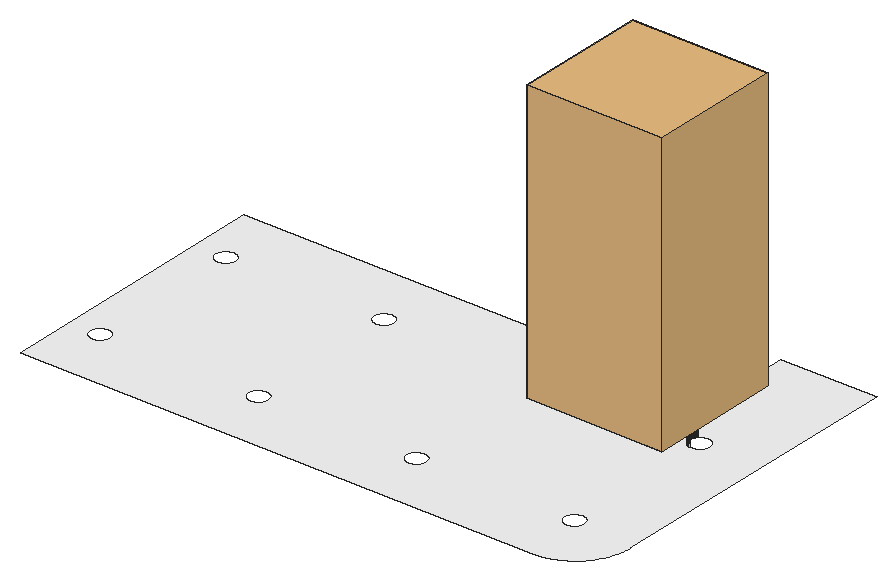
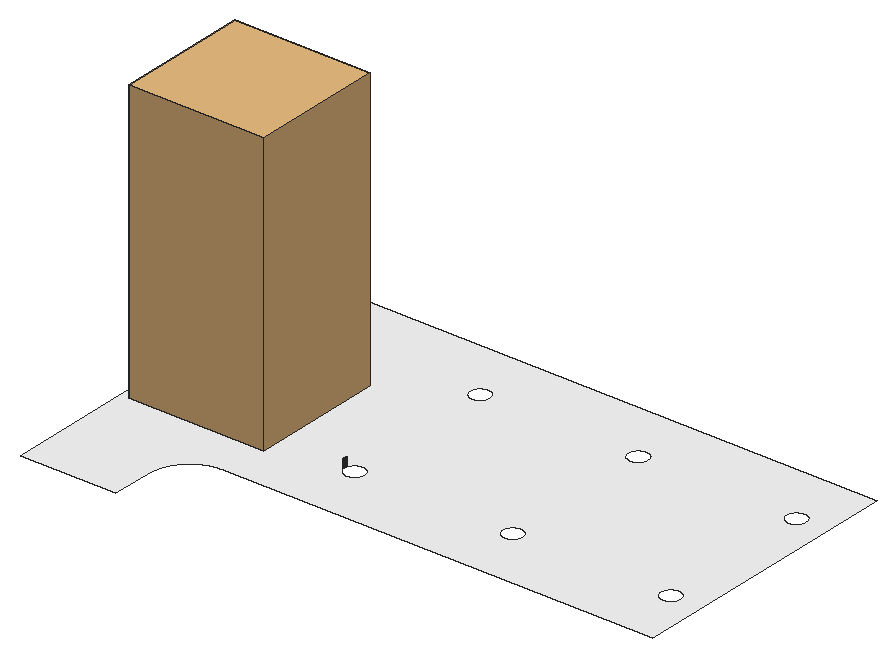
# SketchUp Ruby script. Lengths in inches.
U = 1.inch
M = Sketchup.active_model
def pt(a) = Geom::Point3d.new(a.map { |v| v * U })
def face(e, loops, mat)
  f = e.add_face(loops[0].map { |a| pt(a) })
  loops[1..].each { |l| e.add_face(l.map { |a| pt(a) }).erase! }
  f.material = f.back_material = mat if mat
  f
end
# faces: each face lists its corners as indices into pts; further lists are holes
def faces(e, pts, list, mat = nil) = list.each { |f| face(e, (f[0].is_a?(Array) ? f : [f]).map { |l| l.map { |i| pts[i] } }, mat) }
# xy, xz, yz: faces in a plane at the given z, y or x. An outline is a flat list of corners, or four numbers for a rectangle; further outlines are holes
def ring(l) = l.size == 4 ? [[l[0], l[1]], [l[2], l[1]], [l[2], l[3]], [l[0], l[3]]] : l.each_slice(2).to_a
def flat(e, list, mat, &to3) = list.each { |f| face(e, (f[0].is_a?(Array) ? f : [f]).map { |l| ring(l).map { |u, v| to3.(u, v) } }, mat) }
def xy(e, z, list, mat = nil) = flat(e, list, mat) { |x, y| [x, y, z] }
def xz(e, y, list, mat = nil) = flat(e, list, mat) { |x, z| [x, y, z] }
def yz(e, x, list, mat = nil) = flat(e, list, mat) { |y, z| [x, y, z] }
def lines(e, pts, list) = list.each { |a, b| e.add_line(pt(pts[a]), pt(pts[b])) }
# prism: a flat outline (further loops are holes) pulled along v
def prism(e, loops, v, mat = nil)
  f = face(e, loops, mat); d = Geom::Vector3d.new(v.map { |x| x * U })
  f.pushpull(f.normal.samedirection?(d) ? d.length : -d.length)
end
def box(e, o, s, mat = nil) = prism(e, [[o, [o[0] + s[0], o[1], o[2]], [o[0] + s[0], o[1] + s[1], o[2]], [o[0], o[1] + s[1], o[2]]]], [0, 0, s[2]], mat)
def at(x, y, z, deg = 0) = Geom::Transformation.translation(pt([x, y, z])) * Geom::Transformation.rotation(ORIGIN, Z_AXIS, deg.degrees)
def axes(o, x, y, z) = Geom::Transformation.new([*x, 0, *y, 0, *z, 0, *pt(o).to_a, 1])
def part(name) = M.definitions.add(name)
# library, detail: a bought-in or finely detailed component or shape, given as its bounding box
def library(name, o, s) = part(name).tap { |d| box(d.entities, o, s) }
def detail(e, o, s) = box(e.add_group.entities, o, s)
def put(e, d, t, mat = nil) = e.add_instance(d, t).tap { |i| i.material = mat if mat }
def group(e, t, mat = nil) = e.add_group.tap { |g| g.transformation = t; g.material = mat if mat }.entities
root = M.entities
M.materials.add("[Quartz Light Grey]").color = [251, 251, 252]
c1 = library("aaa (1)",[154.83,121.66,0],[39.67,38.89,82.21])
xy(root,117,[[[60,189,60,271,186.3125,271,186.47,271.01,186.63,271.02,186.78,271.03,187.1,271.05,187.25,271.07,187.41,271.08,187.57,271.1,187.72,271.125,187.88,271.15,188.03,271.17,188.1875,271.2,188.34,271.23,188.49,271.26,188.65,271.3,188.8,271.33,188.95,271.37,189.11,271.41,189.41,271.49,189.86,271.64,190.01,271.6875,190.15,271.74,190.3,271.8,190.45,271.85,190.59,271.91,190.74,271.97,190.88,272.04,191.02,272.1,191.17,272.17,191.73,272.45,191.86,272.53,192,272.61,192.14,272.6875,192.27,272.77,192.4,272.85,192.54,272.9375,192.67,273.02,192.93,273.2,193.05,273.29,193.18,273.38,193.31,273.48,193.43,273.58,193.55,273.67,193.67,273.77,193.91,273.98,194.03,274.08,194.15,274.1875,194.26,274.3,194.375,274.4,194.49,274.51,194.6,274.625,194.7,274.74,194.8125,274.85,194.92,274.97,195.02,275.09,195.23,275.33,195.33,275.45,195.42,275.57,195.52,275.69,195.62,275.82,195.71,275.95,195.8,276.07,195.98,276.33,196.0625,276.46,196.15,276.6,196.23,276.73,196.3125,276.86,196.39,277,196.47,277.14,196.55,277.27,196.83,277.83,196.9,277.98,196.96,278.12,197.03,278.26,197.09,278.41,197.15,278.55,197.2,278.7,197.26,278.85,197.3125,278.99,197.36,279.14,197.51,279.59,197.59,279.89,197.63,280.05,197.67,280.2,197.7,280.35,197.74,280.51,197.77,280.66,197.8,280.8125,197.83,280.97,197.85,281.12,197.875,281.28,197.9,281.43,197.92,281.59,197.93,281.75,197.95,281.9,197.97,282.22,197.98,282.37,197.99,282.53,198,282.6875,198,295,226,295,226,204.79,225.99,204.58,225.99,204.37,225.97,203.95,225.95,203.74,225.93,203.54,225.89,203.12,225.83,202.7,225.8,202.5,225.77,202.29,225.73,202.08,225.69,201.88,225.65,201.67,225.61,201.47,225.56,201.26,225.51,201.0625,225.45,200.86,225.4,200.66,225.22,200.06,225.01,199.46,224.9375,199.27,224.86,199.07,224.78,198.88,224.7,198.68,224.62,198.49,224.35,197.92,224.26,197.74,224.16,197.55,224.0625,197.37,223.96,197.18,223.86,197,223.53,196.46,223.42,196.29,223.3,196.11,223.1875,195.9375,223.07,195.77,222.94,195.6,222.82,195.43,222.69,195.26,222.57,195.09,222.43,194.93,222.17,194.61,221.89,194.29,221.61,193.99,221.46,193.84,221.3125,193.6875,221.16,193.54,221.01,193.39,220.71,193.11,220.39,192.83,220.07,192.57,219.91,192.43,219.74,192.31,219.57,192.18,219.4,192.06,219.23,191.93,219.0625,191.8125,218.89,191.7,218.71,191.58,218.54,191.47,218,191.14,217.82,191.04,217.63,190.9375,217.45,190.84,217.26,190.74,217.08,190.65,216.51,190.38,216.32,190.3,216.12,190.22,215.93,190.14,215.73,190.0625,215.54,189.99,214.94,189.78,214.34,189.6,214.14,189.55,213.9375,189.49,213.74,189.44,213.53,189.39,213.33,189.35,213.12,189.31,212.92,189.27,212.71,189.23,212.5,189.2,212.3,189.17,211.88,189.11,211.46,189.07,211.26,189.05,211.05,189.03,210.63,189.01,210.42,189.01,210.21,189],[68.84,204,69.16,204,69.24,204.01,69.3125,204.02,69.39,204.03,69.55,204.05,69.625,204.07,69.7,204.08,69.78,204.1,69.85,204.125,69.93,204.15,70,204.17,70.08,204.2,70.29,204.29,70.36,204.33,70.43,204.36,70.57,204.44,70.63,204.48,70.7,204.53,70.76,204.57,70.83,204.62,71.07,204.82,71.12,204.88,71.18,204.93,71.38,205.17,71.43,205.24,71.47,205.3,71.52,205.37,71.56,205.43,71.64,205.57,71.67,205.64,71.71,205.71,71.8,205.92,71.83,206,71.85,206.07,71.875,206.15,71.9,206.22,71.92,206.3,71.93,206.375,71.95,206.45,71.97,206.61,71.98,206.6875,71.99,206.76,72,206.84,72,207.16,71.99,207.24,71.98,207.3125,71.97,207.39,71.95,207.55,71.93,207.625,71.92,207.7,71.9,207.78,71.875,207.85,71.85,207.93,71.83,208,71.8,208.08,71.71,208.29,71.67,208.36,71.64,208.43,71.56,208.57,71.52,208.63,71.47,208.7,71.43,208.76,71.38,208.83,71.18,209.07,71.12,209.12,71.07,209.18,70.83,209.38,70.76,209.43,70.7,209.47,70.63,209.52,70.57,209.56,70.43,209.64,70.36,209.67,70.29,209.71,70.08,209.8,70,209.83,69.93,209.85,69.85,209.875,69.78,209.9,69.7,209.92,69.625,209.93,69.55,209.95,69.39,209.97,69.3125,209.98,69.24,209.99,69.16,210,68.84,210,68.76,209.99,68.6875,209.98,68.61,209.97,68.45,209.95,68.375,209.93,68.3,209.92,68.22,209.9,68.15,209.875,68.07,209.85,68,209.83,67.92,209.8,67.71,209.71,67.64,209.67,67.57,209.64,67.43,209.56,67.37,209.52,67.3,209.47,67.24,209.43,67.17,209.38,66.93,209.18,66.88,209.12,66.82,209.07,66.62,208.83,66.57,208.76,66.53,208.7,66.48,208.63,66.44,208.57,66.36,208.43,66.33,208.36,66.29,208.29,66.2,208.08,66.17,208,66.15,207.93,66.125,207.85,66.1,207.78,66.08,207.7,66.07,207.625,66.05,207.55,66.03,207.39,66.02,207.3125,66.01,207.24,66,207.16,66,206.84,66.01,206.76,66.02,206.6875,66.03,206.61,66.05,206.45,66.07,206.375,66.08,206.3,66.1,206.22,66.125,206.15,66.15,206.07,66.17,206,66.2,205.92,66.29,205.71,66.33,205.64,66.36,205.57,66.44,205.43,66.48,205.37,66.53,205.3,66.57,205.24,66.62,205.17,66.82,204.93,66.88,204.88,66.93,204.82,67.17,204.62,67.24,204.57,67.3,204.53,67.37,204.48,67.43,204.44,67.57,204.36,67.64,204.33,67.71,204.29,67.92,204.2,68,204.17,68.07,204.15,68.15,204.125,68.22,204.1,68.3,204.08,68.375,204.07,68.45,204.05,68.61,204.03,68.6875,204.02,68.76,204.01],[68.84,250,69.16,250,69.24,250.01,69.3125,250.02,69.39,250.03,69.55,250.05,69.625,250.07,69.7,250.08,69.78,250.1,69.85,250.125,69.93,250.15,70,250.17,70.08,250.2,70.29,250.29,70.36,250.33,70.43,250.36,70.57,250.44,70.63,250.48,70.7,250.53,70.76,250.57,70.83,250.62,71.07,250.82,71.12,250.88,71.18,250.93,71.38,251.17,71.43,251.24,71.47,251.3,71.52,251.37,71.56,251.43,71.64,251.57,71.67,251.64,71.71,251.71,71.8,251.92,71.83,252,71.85,252.07,71.875,252.15,71.9,252.22,71.92,252.3,71.93,252.375,71.95,252.45,71.97,252.61,71.98,252.6875,71.99,252.76,72,252.84,72,253.16,71.99,253.24,71.98,253.3125,71.97,253.39,71.95,253.55,71.93,253.625,71.92,253.7,71.9,253.78,71.875,253.85,71.85,253.93,71.83,254,71.8,254.08,71.71,254.29,71.67,254.36,71.64,254.43,71.56,254.57,71.52,254.63,71.47,254.7,71.43,254.76,71.38,254.83,71.18,255.07,71.12,255.12,71.07,255.18,70.83,255.38,70.76,255.43,70.7,255.47,70.63,255.52,70.57,255.56,70.43,255.64,70.36,255.67,70.29,255.71,70.08,255.8,70,255.83,69.93,255.85,69.85,255.875,69.78,255.9,69.7,255.92,69.625,255.93,69.55,255.95,69.39,255.97,69.3125,255.98,69.24,255.99,69.16,256,68.84,256,68.76,255.99,68.6875,255.98,68.61,255.97,68.45,255.95,68.375,255.93,68.3,255.92,68.22,255.9,68.15,255.875,68.07,255.85,68,255.83,67.92,255.8,67.71,255.71,67.64,255.67,67.57,255.64,67.43,255.56,67.37,255.52,67.3,255.47,67.24,255.43,67.17,255.38,66.93,255.18,66.88,255.12,66.82,255.07,66.62,254.83,66.57,254.76,66.53,254.7,66.48,254.63,66.44,254.57,66.36,254.43,66.33,254.36,66.29,254.29,66.2,254.08,66.17,254,66.15,253.93,66.125,253.85,66.1,253.78,66.08,253.7,66.07,253.625,66.05,253.55,66.03,253.39,66.02,253.3125,66.01,253.24,66,253.16,66,252.84,66.01,252.76,66.02,252.6875,66.03,252.61,66.05,252.45,66.07,252.375,66.08,252.3,66.1,252.22,66.125,252.15,66.15,252.07,66.17,252,66.2,251.92,66.29,251.71,66.33,251.64,66.36,251.57,66.44,251.43,66.48,251.37,66.53,251.3,66.57,251.24,66.62,251.17,66.82,250.93,66.88,250.88,66.93,250.82,67.17,250.62,67.24,250.57,67.3,250.53,67.37,250.48,67.43,250.44,67.57,250.36,67.64,250.33,67.71,250.29,67.92,250.2,68,250.17,68.07,250.15,68.15,250.125,68.22,250.1,68.3,250.08,68.375,250.07,68.45,250.05,68.61,250.03,68.6875,250.02,68.76,250.01],[207.84,250,208.16,250,208.24,250.01,208.3125,250.02,208.39,250.03,208.55,250.05,208.625,250.07,208.7,250.08,208.78,250.1,208.85,250.125,208.93,250.15,209,250.17,209.08,250.2,209.29,250.29,209.36,250.33,209.43,250.36,209.57,250.44,209.63,250.48,209.7,250.53,209.76,250.57,209.83,250.62,210.07,250.82,210.12,250.88,210.18,250.93,210.38,251.17,210.43,251.24,210.47,251.3,210.52,251.37,210.56,251.43,210.64,251.57,210.67,251.64,210.71,251.71,210.8,251.92,210.83,252,210.85,252.07,210.875,252.15,210.9,252.22,210.92,252.3,210.93,252.375,210.95,252.45,210.97,252.61,210.98,252.6875,210.99,252.76,211,252.84,211,253.16,210.99,253.24,210.98,253.3125,210.97,253.39,210.95,253.55,210.93,253.625,210.92,253.7,210.9,253.78,210.875,253.85,210.85,253.93,210.83,254,210.8,254.08,210.71,254.29,210.67,254.36,210.64,254.43,210.56,254.57,210.52,254.63,210.47,254.7,210.43,254.76,210.38,254.83,210.18,255.07,210.12,255.12,210.07,255.18,209.83,255.38,209.76,255.43,209.7,255.47,209.63,255.52,209.57,255.56,209.43,255.64,209.36,255.67,209.29,255.71,209.08,255.8,209,255.83,208.93,255.85,208.85,255.875,208.78,255.9,208.7,255.92,208.625,255.93,208.55,255.95,208.39,255.97,208.3125,255.98,208.24,255.99,208.16,256,207.84,256,207.76,255.99,207.6875,255.98,207.61,255.97,207.45,255.95,207.375,255.93,207.3,255.92,207.22,255.9,207.15,255.875,207.07,255.85,207,255.83,206.92,255.8,206.71,255.71,206.64,255.67,206.57,255.64,206.43,255.56,206.37,255.52,206.3,255.47,206.24,255.43,206.17,255.38,205.93,255.18,205.88,255.12,205.82,255.07,205.62,254.83,205.57,254.76,205.53,254.7,205.48,254.63,205.44,254.57,205.36,254.43,205.33,254.36,205.29,254.29,205.2,254.08,205.17,254,205.15,253.93,205.125,253.85,205.1,253.78,205.08,253.7,205.07,253.625,205.05,253.55,205.03,253.39,205.02,253.3125,205.01,253.24,205,253.16,205,252.84,205.01,252.76,205.02,252.6875,205.03,252.61,205.05,252.45,205.07,252.375,205.08,252.3,205.1,252.22,205.125,252.15,205.15,252.07,205.17,252,205.2,251.92,205.29,251.71,205.33,251.64,205.36,251.57,205.44,251.43,205.48,251.37,205.53,251.3,205.57,251.24,205.62,251.17,205.82,250.93,205.88,250.88,205.93,250.82,206.17,250.62,206.24,250.57,206.3,250.53,206.37,250.48,206.43,250.44,206.57,250.36,206.64,250.33,206.71,250.29,206.92,250.2,207,250.17,207.07,250.15,207.15,250.125,207.22,250.1,207.3,250.08,207.375,250.07,207.45,250.05,207.61,250.03,207.6875,250.02,207.76,250.01],[207.84,204,208.16,204,208.24,204.01,208.3125,204.02,208.39,204.03,208.55,204.05,208.625,204.07,208.7,204.08,208.78,204.1,208.85,204.125,208.93,204.15,209,204.17,209.08,204.2,209.29,204.29,209.36,204.33,209.43,204.36,209.57,204.44,209.63,204.48,209.7,204.53,209.76,204.57,209.83,204.62,210.07,204.82,210.12,204.88,210.18,204.93,210.38,205.17,210.43,205.24,210.47,205.3,210.52,205.37,210.56,205.43,210.64,205.57,210.67,205.64,210.71,205.71,210.8,205.92,210.83,206,210.85,206.07,210.875,206.15,210.9,206.22,210.92,206.3,210.93,206.375,210.95,206.45,210.97,206.61,210.98,206.6875,210.99,206.76,211,206.84,211,207.16,210.99,207.24,210.98,207.3125,210.97,207.39,210.95,207.55,210.93,207.625,210.92,207.7,210.9,207.78,210.875,207.85,210.85,207.93,210.83,208,210.8,208.08,210.71,208.29,210.67,208.36,210.64,208.43,210.56,208.57,210.52,208.63,210.47,208.7,210.43,208.76,210.38,208.83,210.18,209.07,210.12,209.12,210.07,209.18,209.83,209.38,209.76,209.43,209.7,209.47,209.63,209.52,209.57,209.56,209.43,209.64,209.36,209.67,209.29,209.71,209.08,209.8,209,209.83,208.93,209.85,208.85,209.875,208.78,209.9,208.7,209.92,208.625,209.93,208.55,209.95,208.39,209.97,208.3125,209.98,208.24,209.99,208.16,210,207.84,210,207.76,209.99,207.6875,209.98,207.61,209.97,207.45,209.95,207.375,209.93,207.3,209.92,207.22,209.9,207.15,209.875,207.07,209.85,207,209.83,206.92,209.8,206.71,209.71,206.64,209.67,206.57,209.64,206.43,209.56,206.37,209.52,206.3,209.47,206.24,209.43,206.17,209.38,205.93,209.18,205.88,209.12,205.82,209.07,205.62,208.83,205.57,208.76,205.53,208.7,205.48,208.63,205.44,208.57,205.36,208.43,205.33,208.36,205.29,208.29,205.2,208.08,205.17,208,205.15,207.93,205.125,207.85,205.1,207.78,205.08,207.7,205.07,207.625,205.05,207.55,205.03,207.39,205.02,207.3125,205.01,207.24,205,207.16,205,206.84,205.01,206.76,205.02,206.6875,205.03,206.61,205.05,206.45,205.07,206.375,205.08,206.3,205.1,206.22,205.125,206.15,205.15,206.07,205.17,206,205.2,205.92,205.29,205.71,205.33,205.64,205.36,205.57,205.44,205.43,205.48,205.37,205.53,205.3,205.57,205.24,205.62,205.17,205.82,204.93,205.88,204.88,205.93,204.82,206.17,204.62,206.24,204.57,206.3,204.53,206.37,204.48,206.43,204.44,206.57,204.36,206.64,204.33,206.71,204.29,206.92,204.2,207,204.17,207.07,204.15,207.15,204.125,207.22,204.1,207.3,204.08,207.375,204.07,207.45,204.05,207.61,204.03,207.6875,204.02,207.76,204.01],[115.18,250,115.49,250,115.65,250.02,115.72,250.03,115.88,250.05,115.96,250.07,116.03,250.08,116.11,250.1,116.19,250.125,116.26,250.15,116.33,250.17,116.41,250.2,116.55,250.26,116.625,250.29,116.7,250.33,116.76,250.36,116.97,250.48,117.03,250.53,117.1,250.57,117.4,250.82,117.45,250.88,117.51,250.93,117.5625,250.99,117.61,251.05,117.71,251.17,117.76,251.24,117.81,251.3,117.85,251.37,117.89,251.43,118.01,251.64,118.13,251.92,118.16,252,118.1875,252.07,118.21,252.15,118.23,252.22,118.25,252.3,118.27,252.375,118.28,252.45,118.3,252.53,118.31,252.61,118.32,252.6875,118.32,252.76,118.33,252.84,118.33,253.16,118.32,253.24,118.32,253.3125,118.31,253.39,118.3,253.47,118.28,253.55,118.27,253.625,118.25,253.7,118.23,253.78,118.21,253.85,118.1875,253.93,118.16,254,118.13,254.08,118.01,254.36,117.89,254.57,117.85,254.63,117.81,254.7,117.76,254.76,117.71,254.83,117.61,254.95,117.5625,255.01,117.51,255.07,117.45,255.12,117.4,255.18,117.1,255.43,117.03,255.47,116.97,255.52,116.76,255.64,116.7,255.67,116.625,255.71,116.55,255.74,116.41,255.8,116.33,255.83,116.26,255.85,116.19,255.875,116.11,255.9,116.03,255.92,115.96,255.93,115.88,255.95,115.72,255.97,115.65,255.98,115.49,256,115.18,256,114.86,255.96,114.79,255.95,114.71,255.93,114.63,255.92,114.56,255.9,114.48,255.875,114.41,255.85,114.33,255.83,114.19,255.77,114.11,255.74,114.04,255.71,113.97,255.67,113.9,255.64,113.83,255.6,113.77,255.56,113.7,255.52,113.63,255.47,113.57,255.43,113.45,255.33,113.38,255.28,113.33,255.23,113.27,255.18,113.1,255.01,112.95,254.83,112.91,254.76,112.86,254.7,112.82,254.63,112.78,254.57,112.66,254.36,112.59,254.22,112.5625,254.15,112.53,254.08,112.51,254,112.48,253.93,112.46,253.85,112.4375,253.78,112.42,253.7,112.38,253.55,112.36,253.39,112.35,253.3125,112.34,253.24,112.34,253.16,112.33,253.08,112.33,252.92,112.34,252.84,112.34,252.76,112.35,252.6875,112.36,252.61,112.38,252.45,112.42,252.3,112.4375,252.22,112.46,252.15,112.48,252.07,112.51,252,112.53,251.92,112.5625,251.85,112.59,251.78,112.66,251.64,112.78,251.43,112.82,251.37,112.86,251.3,112.91,251.24,112.95,251.17,113.1,250.99,113.27,250.82,113.33,250.77,113.38,250.72,113.45,250.67,113.57,250.57,113.63,250.53,113.7,250.48,113.77,250.44,113.83,250.4,113.9,250.36,113.97,250.33,114.04,250.29,114.11,250.26,114.19,250.23,114.33,250.17,114.41,250.15,114.48,250.125,114.56,250.1,114.63,250.08,114.71,250.07,114.79,250.05,114.86,250.04],[115.18,204,115.49,204,115.65,204.02,115.72,204.03,115.88,204.05,115.96,204.07,116.03,204.08,116.11,204.1,116.19,204.125,116.26,204.15,116.33,204.17,116.41,204.2,116.55,204.26,116.625,204.29,116.7,204.33,116.76,204.36,116.97,204.48,117.03,204.53,117.1,204.57,117.4,204.82,117.45,204.88,117.51,204.93,117.5625,204.99,117.61,205.05,117.71,205.17,117.76,205.24,117.81,205.3,117.85,205.37,117.89,205.43,118.01,205.64,118.13,205.92,118.16,206,118.1875,206.07,118.21,206.15,118.23,206.22,118.25,206.3,118.27,206.375,118.28,206.45,118.3,206.53,118.31,206.61,118.32,206.6875,118.32,206.76,118.33,206.84,118.33,207.16,118.32,207.24,118.32,207.3125,118.31,207.39,118.3,207.47,118.28,207.55,118.27,207.625,118.25,207.7,118.23,207.78,118.21,207.85,118.1875,207.93,118.16,208,118.13,208.08,118.01,208.36,117.89,208.57,117.85,208.63,117.81,208.7,117.76,208.76,117.71,208.83,117.61,208.95,117.5625,209.01,117.51,209.07,117.45,209.12,117.4,209.18,117.1,209.43,117.03,209.47,116.97,209.52,116.76,209.64,116.7,209.67,116.625,209.71,116.55,209.74,116.41,209.8,116.33,209.83,116.26,209.85,116.19,209.875,116.11,209.9,116.03,209.92,115.96,209.93,115.88,209.95,115.72,209.97,115.65,209.98,115.49,210,115.18,210,114.86,209.96,114.79,209.95,114.71,209.93,114.63,209.92,114.56,209.9,114.48,209.875,114.41,209.85,114.33,209.83,114.19,209.77,114.11,209.74,114.04,209.71,113.97,209.67,113.9,209.64,113.83,209.6,113.77,209.56,113.7,209.52,113.63,209.47,113.57,209.43,113.45,209.33,113.38,209.28,113.33,209.23,113.27,209.18,113.1,209.01,112.95,208.83,112.91,208.76,112.86,208.7,112.82,208.63,112.78,208.57,112.66,208.36,112.59,208.22,112.5625,208.15,112.53,208.08,112.51,208,112.48,207.93,112.46,207.85,112.4375,207.78,112.42,207.7,112.38,207.55,112.36,207.39,112.35,207.3125,112.34,207.24,112.34,207.16,112.33,207.08,112.33,206.92,112.34,206.84,112.34,206.76,112.35,206.6875,112.36,206.61,112.38,206.45,112.42,206.3,112.4375,206.22,112.46,206.15,112.48,206.07,112.51,206,112.53,205.92,112.5625,205.85,112.59,205.78,112.66,205.64,112.78,205.43,112.82,205.37,112.86,205.3,112.91,205.24,112.95,205.17,113.1,204.99,113.27,204.82,113.33,204.77,113.38,204.72,113.45,204.67,113.57,204.57,113.63,204.53,113.7,204.48,113.77,204.44,113.83,204.4,113.9,204.36,113.97,204.33,114.04,204.29,114.11,204.26,114.19,204.23,114.33,204.17,114.41,204.15,114.48,204.125,114.56,204.1,114.63,204.08,114.71,204.07,114.79,204.05,114.86,204.04],[161.51,250,161.82,250,162.14,250.04,162.21,250.05,162.29,250.07,162.37,250.08,162.44,250.1,162.52,250.125,162.59,250.15,162.67,250.17,162.81,250.23,162.89,250.26,162.96,250.29,163.03,250.33,163.1,250.36,163.17,250.4,163.23,250.44,163.3,250.48,163.37,250.53,163.43,250.57,163.55,250.67,163.62,250.72,163.67,250.77,163.73,250.82,163.9,250.99,164.05,251.17,164.09,251.24,164.14,251.3,164.18,251.37,164.22,251.43,164.34,251.64,164.41,251.78,164.4375,251.85,164.47,251.92,164.49,252,164.52,252.07,164.54,252.15,164.5625,252.22,164.58,252.3,164.62,252.45,164.64,252.61,164.65,252.6875,164.66,252.76,164.66,252.84,164.67,252.92,164.67,253.08,164.66,253.16,164.66,253.24,164.65,253.3125,164.64,253.39,164.62,253.55,164.58,253.7,164.5625,253.78,164.54,253.85,164.52,253.93,164.49,254,164.47,254.08,164.4375,254.15,164.41,254.22,164.34,254.36,164.22,254.57,164.18,254.63,164.14,254.7,164.09,254.76,164.05,254.83,163.9,255.01,163.73,255.18,163.67,255.23,163.62,255.28,163.55,255.33,163.43,255.43,163.37,255.47,163.3,255.52,163.23,255.56,163.17,255.6,163.1,255.64,163.03,255.67,162.96,255.71,162.89,255.74,162.81,255.77,162.67,255.83,162.59,255.85,162.52,255.875,162.44,255.9,162.37,255.92,162.29,255.93,162.21,255.95,162.14,255.96,161.82,256,161.51,256,161.35,255.98,161.28,255.97,161.12,255.95,161.04,255.93,160.97,255.92,160.89,255.9,160.81,255.875,160.74,255.85,160.67,255.83,160.59,255.8,160.45,255.74,160.375,255.71,160.3,255.67,160.24,255.64,160.03,255.52,159.97,255.47,159.9,255.43,159.6,255.18,159.55,255.12,159.49,255.07,159.4375,255.01,159.39,254.95,159.29,254.83,159.24,254.76,159.19,254.7,159.15,254.63,159.11,254.57,158.99,254.36,158.87,254.08,158.84,254,158.8125,253.93,158.79,253.85,158.77,253.78,158.75,253.7,158.73,253.625,158.72,253.55,158.7,253.47,158.69,253.39,158.68,253.3125,158.68,253.24,158.67,253.16,158.67,252.84,158.68,252.76,158.68,252.6875,158.69,252.61,158.7,252.53,158.72,252.45,158.73,252.375,158.75,252.3,158.77,252.22,158.79,252.15,158.8125,252.07,158.84,252,158.87,251.92,158.99,251.64,159.11,251.43,159.15,251.37,159.19,251.3,159.24,251.24,159.29,251.17,159.39,251.05,159.4375,250.99,159.49,250.93,159.55,250.88,159.6,250.82,159.9,250.57,159.97,250.53,160.03,250.48,160.24,250.36,160.3,250.33,160.375,250.29,160.45,250.26,160.59,250.2,160.67,250.17,160.74,250.15,160.81,250.125,160.89,250.1,160.97,250.08,161.04,250.07,161.12,250.05,161.28,250.03,161.35,250.02],[161.51,204,161.82,204,162.14,204.04,162.21,204.05,162.29,204.07,162.37,204.08,162.44,204.1,162.52,204.125,162.59,204.15,162.67,204.17,162.81,204.23,162.89,204.26,162.96,204.29,163.03,204.33,163.1,204.36,163.17,204.4,163.23,204.44,163.3,204.48,163.37,204.53,163.43,204.57,163.55,204.67,163.62,204.72,163.67,204.77,163.73,204.82,163.9,204.99,164.05,205.17,164.09,205.24,164.14,205.3,164.18,205.37,164.22,205.43,164.34,205.64,164.41,205.78,164.4375,205.85,164.47,205.92,164.49,206,164.52,206.07,164.54,206.15,164.5625,206.22,164.58,206.3,164.62,206.45,164.64,206.61,164.65,206.6875,164.66,206.76,164.66,206.84,164.67,206.92,164.67,207.08,164.66,207.16,164.66,207.24,164.65,207.3125,164.64,207.39,164.62,207.55,164.58,207.7,164.5625,207.78,164.54,207.85,164.52,207.93,164.49,208,164.47,208.08,164.4375,208.15,164.41,208.22,164.34,208.36,164.22,208.57,164.18,208.63,164.14,208.7,164.09,208.76,164.05,208.83,163.9,209.01,163.73,209.18,163.67,209.23,163.62,209.28,163.55,209.33,163.43,209.43,163.37,209.47,163.3,209.52,163.23,209.56,163.17,209.6,163.1,209.64,163.03,209.67,162.96,209.71,162.89,209.74,162.81,209.77,162.67,209.83,162.59,209.85,162.52,209.875,162.44,209.9,162.37,209.92,162.29,209.93,162.21,209.95,162.14,209.96,161.82,210,161.51,210,161.35,209.98,161.28,209.97,161.12,209.95,161.04,209.93,160.97,209.92,160.89,209.9,160.81,209.875,160.74,209.85,160.67,209.83,160.59,209.8,160.45,209.74,160.375,209.71,160.3,209.67,160.24,209.64,160.03,209.52,159.97,209.47,159.9,209.43,159.6,209.18,159.55,209.12,159.49,209.07,159.4375,209.01,159.39,208.95,159.29,208.83,159.24,208.76,159.19,208.7,159.15,208.63,159.11,208.57,158.99,208.36,158.87,208.08,158.84,208,158.8125,207.93,158.79,207.85,158.77,207.78,158.75,207.7,158.73,207.625,158.72,207.55,158.7,207.47,158.69,207.39,158.68,207.3125,158.68,207.24,158.67,207.16,158.67,206.84,158.68,206.76,158.68,206.6875,158.69,206.61,158.7,206.53,158.72,206.45,158.73,206.375,158.75,206.3,158.77,206.22,158.79,206.15,158.8125,206.07,158.84,206,158.87,205.92,158.99,205.64,159.11,205.43,159.15,205.37,159.19,205.3,159.24,205.24,159.29,205.17,159.39,205.05,159.4375,204.99,159.49,204.93,159.55,204.88,159.6,204.82,159.9,204.57,159.97,204.53,160.03,204.48,160.24,204.36,160.3,204.33,160.375,204.29,160.45,204.26,160.59,204.2,160.67,204.17,160.74,204.15,160.81,204.125,160.89,204.1,160.97,204.08,161.04,204.07,161.12,204.05,161.28,204.03,161.35,204.02]]],"[Quartz Light Grey]")
yz(root,164.66,[[252.76,117,252.84,119.5],[253.16,117,253.24,119.5]],"[Quartz Light Grey]")
yz(root,164.67,[[252.92,117,253,119.5],[253,117,253.08,119.5]],"[Quartz Light Grey]")
yz(root,205,[[252.84,117,252.92,119.5],[252.92,117,253,119.5],[253,117,253.08,119.5],[253.08,117,253.16,119.5]],"[Quartz Light Grey]")
p = [[207.07,250.15,117],[207,250.17,117],[207,250.17,119.5],[207.07,250.15,119.5],[207.15,250.125,117],[207.15,250.125,119.5],
  [207.22,250.1,117],[207.22,250.1,119.5],[206.85,250.23,117],[206.78,250.26,117],[206.78,250.26,119.5],[206.85,250.23,119.5],
  [206.92,250.2,117],[206.92,250.2,119.5],[206.64,250.33,117],[206.57,250.36,117],[206.57,250.36,119.5],[206.64,250.33,119.5],
  [206.71,250.29,117],[206.71,250.29,119.5],[206.43,250.44,117],[206.37,250.48,117],[206.37,250.48,119.5],[206.43,250.44,119.5],
  [206.5,250.4,117],[206.5,250.4,119.5],[206.3,250.53,117],[206.24,250.57,117],[206.24,250.57,119.5],[206.3,250.53,119.5],
  [206.17,250.62,117],[206.11,250.67,117],[206.11,250.67,119.5],[206.17,250.62,119.5],[206.05,250.72,117],[205.99,250.77,117],
  [205.99,250.77,119.5],[206.05,250.72,119.5],[205.93,250.82,117],[205.88,250.88,117],[205.88,250.88,119.5],[205.93,250.82,119.5],
  [205.82,250.93,117],[205.77,250.99,117],[205.77,250.99,119.5],[205.82,250.93,119.5],[205.72,251.05,117],[205.72,251.05,119.5],
  [205.67,251.11,117],[205.62,251.17,117],[205.62,251.17,119.5],[205.67,251.11,119.5],[205.57,251.24,117],[205.53,251.3,117],
  [205.53,251.3,119.5],[205.57,251.24,119.5],[205.48,251.37,117],[205.48,251.37,119.5],[205.44,251.43,117],[205.4,251.5,117],
  [205.4,251.5,119.5],[205.44,251.43,119.5],[205.36,251.57,117],[205.36,251.57,119.5],[205.33,251.64,117],[205.29,251.71,117],
  [205.29,251.71,119.5],[205.33,251.64,119.5],[205.26,251.78,117],[205.26,251.78,119.5],[205.23,251.85,117],[205.23,251.85,119.5],
  [205.2,251.92,117],[205.17,252,117],[205.17,252,119.5],[205.2,251.92,119.5],[205.15,252.07,117],[205.15,252.07,119.5],
  [205.125,252.15,117],[205.1,252.22,117],[205.1,252.22,119.5],[205.125,252.15,119.5],[164.58,252.3,117],[164.5625,252.22,117],
  [164.5625,252.22,119.5],[164.58,252.3,119.5],[205.08,252.3,117],[205.08,252.3,119.5],[164.6,252.375,117],[164.6,252.375,119.5],
  [205.07,252.375,117],[205.07,252.375,119.5],[164.62,252.45,117],[164.62,252.45,119.5],[205.05,252.45,117],[205.05,252.45,119.5],
  [164.63,252.53,117],[164.63,252.53,119.5],[164.64,252.61,117],[164.64,252.61,119.5],[205.04,252.53,117],[205.03,252.61,117],
  [205.03,252.61,119.5],[205.04,252.53,119.5],[164.65,252.6875,117],[164.65,252.6875,119.5],[205.02,252.6875,117],[205.02,252.6875,119.5],
  [164.66,252.76,117],[164.66,252.76,119.5],[205.01,252.76,117],[205.01,252.76,119.5],[164.67,252.92,117],[164.66,252.84,117],
  [164.66,252.84,119.5],[164.67,252.92,119.5],[205,252.84,117],[205,252.84,119.5],[164.66,253.16,117],[164.67,253.08,117],
  [164.67,253.08,119.5],[164.66,253.16,119.5],[164.65,253.3125,117],[164.66,253.24,117],[164.66,253.24,119.5],[164.65,253.3125,119.5],
  [205,253.16,117],[205.01,253.24,117],[205.01,253.24,119.5],[205,253.16,119.5],[205.02,253.3125,117],[205.02,253.3125,119.5],
  [164.64,253.39,117],[164.64,253.39,119.5],[205.03,253.39,117],[205.03,253.39,119.5],[164.63,253.47,117],[164.63,253.47,119.5],
  [205.04,253.47,117],[205.04,253.47,119.5],[164.6,253.625,117],[164.62,253.55,117],[164.62,253.55,119.5],[164.6,253.625,119.5],
  [205.05,253.55,117],[205.05,253.55,119.5],[205.07,253.625,117],[205.07,253.625,119.5],[164.58,253.7,117],[164.58,253.7,119.5],
  [205.08,253.7,117],[205.08,253.7,119.5],[164.5625,253.78,117],[164.5625,253.78,119.5],[205.1,253.78,117],[205.1,253.78,119.5],
  [164.54,253.85,117],[164.54,253.85,119.5],[205.125,253.85,117],[205.125,253.85,119.5],[205.15,253.93,117],[205.15,253.93,119.5],
  [205.17,254,117],[205.17,254,119.5],[205.2,254.08,117],[205.2,254.08,119.5],[205.23,254.15,117],[205.23,254.15,119.5],
  [205.26,254.22,117],[205.26,254.22,119.5],[205.29,254.29,117],[205.29,254.29,119.5],[205.33,254.36,117],[205.33,254.36,119.5],
  [205.36,254.43,117],[205.36,254.43,119.5],[205.4,254.5,117],[205.4,254.5,119.5],[205.44,254.57,117],[205.44,254.57,119.5],
  [205.48,254.63,117],[205.48,254.63,119.5],[205.53,254.7,117],[205.53,254.7,119.5],[205.57,254.76,117],[205.57,254.76,119.5],
  [205.62,254.83,117],[205.62,254.83,119.5],[205.67,254.89,117],[205.67,254.89,119.5]]
faces(root,p,[[0,1,2,3],[4,0,3,5],[6,4,5,7],[8,9,10,11],[12,8,11,13],[1,12,13,2],[14,15,16,17],[18,14,17,19],
  [9,18,19,10],[20,21,22,23],[24,20,23,25],[15,24,25,16],[26,27,28,29],[21,26,29,22],[30,31,32,33],[27,30,33,28],
  [34,35,36,37],[31,34,37,32],[38,39,40,41],[35,38,41,36],[42,43,44,45],[39,42,45,40],[43,46,47,44],[48,49,50,51],
  [46,48,51,47],[52,53,54,55],[49,52,55,50],[53,56,57,54],[58,59,60,61],[56,58,61,57],[59,62,63,60],[64,65,66,67],
  [62,64,67,63],[65,68,69,66],[68,70,71,69],[72,73,74,75],[70,72,75,71],[73,76,77,74],[78,79,80,81],[76,78,81,77],
  [82,83,84,85],[79,86,87,80],[88,82,85,89],[86,90,91,87],[92,88,89,93],[90,94,95,91],[96,92,93,97],[98,96,97,99],
  [100,101,102,103],[94,100,103,95],[104,98,99,105],[101,106,107,102],[108,104,105,109],[106,110,111,107],[112,113,114,115],[110,116,117,111],
  [118,119,120,121],[122,123,124,125],[126,127,128,129],[127,130,131,128],[132,122,125,133],[130,134,135,131],[136,132,133,137],[134,138,139,135],
  [140,141,142,143],[141,136,137,142],[138,144,145,139],[144,146,147,145],[148,140,143,149],[146,150,151,147],[152,148,149,153],[150,154,155,151],
  [156,152,153,157],[154,158,159,155],[158,160,161,159],[160,162,163,161],[162,164,165,163],[164,166,167,165],[166,168,169,167],[168,170,171,169],
  [170,172,173,171],[172,174,175,173],[174,176,177,175],[176,178,179,177],[178,180,181,179],[180,182,183,181],[182,184,185,183],[184,186,187,185],
  [186,188,189,187]],"[Quartz Light Grey]")
put(root,c1,at(18.94,110.45,126))
